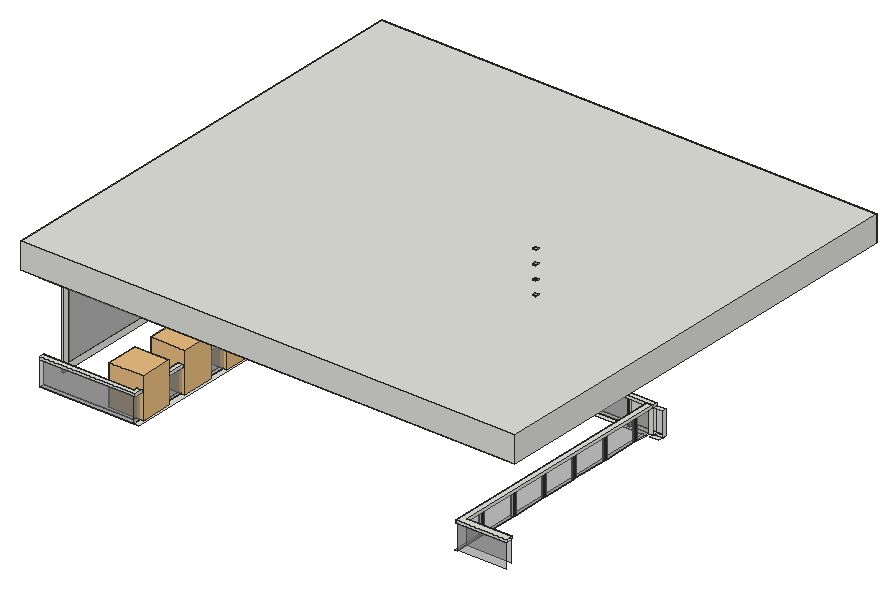
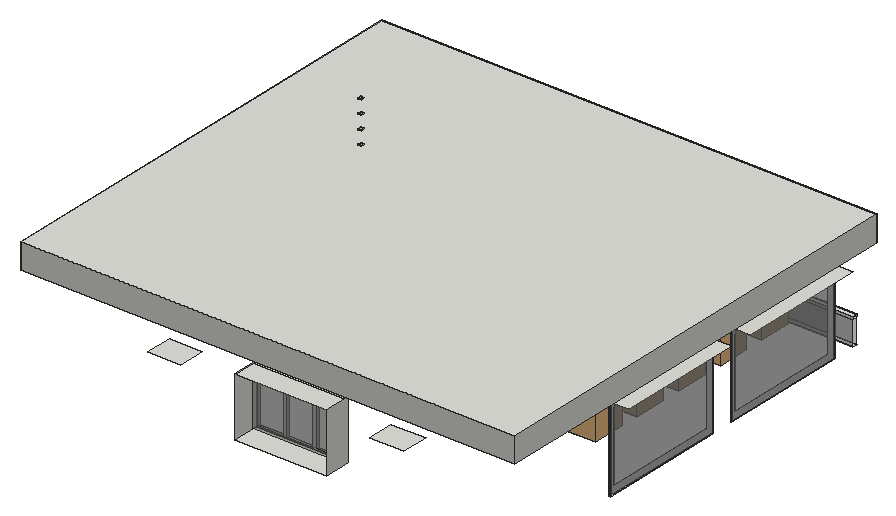
# SketchUp Ruby script. Lengths in inches.
U = 1.inch
M = Sketchup.active_model
def pt(a) = Geom::Point3d.new(a.map { |v| v * U })
def face(e, loops, mat)
  f = e.add_face(loops[0].map { |a| pt(a) })
  loops[1..].each { |l| e.add_face(l.map { |a| pt(a) }).erase! }
  f.material = f.back_material = mat if mat
  f
end
# faces: each face lists its corners as indices into pts; further lists are holes
def faces(e, pts, list, mat = nil) = list.each { |f| face(e, (f[0].is_a?(Array) ? f : [f]).map { |l| l.map { |i| pts[i] } }, mat) }
# xy, xz, yz: faces in a plane at the given z, y or x. An outline is a flat list of corners, or four numbers for a rectangle; further outlines are holes
def ring(l) = l.size == 4 ? [[l[0], l[1]], [l[2], l[1]], [l[2], l[3]], [l[0], l[3]]] : l.each_slice(2).to_a
def flat(e, list, mat, &to3) = list.each { |f| face(e, (f[0].is_a?(Array) ? f : [f]).map { |l| ring(l).map { |u, v| to3.(u, v) } }, mat) }
def xy(e, z, list, mat = nil) = flat(e, list, mat) { |x, y| [x, y, z] }
def xz(e, y, list, mat = nil) = flat(e, list, mat) { |x, z| [x, y, z] }
def yz(e, x, list, mat = nil) = flat(e, list, mat) { |y, z| [x, y, z] }
def lines(e, pts, list) = list.each { |a, b| e.add_line(pt(pts[a]), pt(pts[b])) }
# prism: a flat outline (further loops are holes) pulled along v
def prism(e, loops, v, mat = nil)
  f = face(e, loops, mat); d = Geom::Vector3d.new(v.map { |x| x * U })
  f.pushpull(f.normal.samedirection?(d) ? d.length : -d.length)
end
def box(e, o, s, mat = nil) = prism(e, [[o, [o[0] + s[0], o[1], o[2]], [o[0] + s[0], o[1] + s[1], o[2]], [o[0], o[1] + s[1], o[2]]]], [0, 0, s[2]], mat)
def at(x, y, z, deg = 0) = Geom::Transformation.translation(pt([x, y, z])) * Geom::Transformation.rotation(ORIGIN, Z_AXIS, deg.degrees)
def axes(o, x, y, z) = Geom::Transformation.new([*x, 0, *y, 0, *z, 0, *pt(o).to_a, 1])
def part(name) = M.definitions.add(name)
# library, detail: a bought-in or finely detailed component or shape, given as its bounding box
def library(name, o, s) = part(name).tap { |d| box(d.entities, o, s) }
def detail(e, o, s) = box(e.add_group.entities, o, s)
def put(e, d, t, mat = nil) = e.add_instance(d, t).tap { |i| i.material = mat if mat }
def group(e, t, mat = nil) = e.add_group.tap { |g| g.transformation = t; g.material = mat if mat }.entities
root = M.entities
M.materials.add("Generic").color = [229, 227, 174]
M.materials.add("[Translucent Glass Gray]").color = [128, 128, 128]
M.materials["[Translucent Glass Gray]"].alpha = 0.5
M.materials.add("[Wood Board Cork]").color = [181, 169, 96]
M.materials["[Wood Board Cork]"].alpha = 0.67
c1 = library("Flora+17",[-57.52,158.6,-38.64],[66.99,62.88,77.28])
c2 = part("Group\#2")
xy(c2.entities,0,[[0,0,3,296.5625]])
xy(c2.entities,195.1875,[[0,0,3,296.5625]])
xz(c2.entities,0,[[0,0,3,195.1875]])
xz(c2.entities,296.5625,[[0,0,3,195.1875]])
yz(c2.entities,0,[[0,0,296.5625,195.1875]],"[Translucent Glass Gray]")
yz(c2.entities,3,[[[0,0,296.5625,195.1875],[14.23,14.23,282.34,180.96]]])
yz(c2.entities,3,[[14.23,14.23,282.34,180.96]],"[Translucent Glass Gray]")
c3 = library("Tlon Light 450 Ceiling 152 006",[-8.86,-8.86,-3.78],[17.72,17.72,3.56])
xy(root,231.375,[[45.5625,0,45.5625,11.0625,253.5,11.0625,253.5,562.3125,1038.97,562.3125,1018.75,562.1,1018.84,553.25,966.1875,553.25,966.1875,549.9375,961.1875,549.9375,961.1875,553.25,853.5625,553.25,853.5625,549.9375,848.5625,549.9375,848.5625,553.25,740.9375,553.25,740.9375,549.9375,735.9375,549.9375,735.9375,553.25,609.5,553.25,609.5,549.9375,604.5,549.9375,604.5,553.25,478.0625,553.25,478.0625,549.9375,473.0625,549.9375,473.0625,553.25,346.625,553.25,346.625,549.9375,341.625,549.9375,341.625,553.25,261.0625,553.25,261.0625,512.6,264.375,512.6,264.375,506.23,261.0625,506.23,261.0625,386.1875,264.375,386.1875,264.375,379.8125,261.0625,379.8125,261.0625,279.4375,264.375,279.4375,264.375,273.0625,261.0625,273.0625,261.0625,172.6875,264.375,172.6875,264.375,166.3125,261.0625,166.3125,261.0625,65.9375,264.375,65.9375,264.375,59.5625,261.0625,59.5625,261.0625,0],[261.0625,0,261.0625,59.5625,264.375,59.5625,264.375,65.9375,261.0625,65.9375,261.0625,166.3125,264.375,166.3125,264.375,172.6875,261.0625,172.6875,261.0625,273.0625,264.375,273.0625,264.375,279.4375,261.0625,279.4375,261.0625,379.8125,264.375,379.8125,264.375,386.1875,261.0625,386.1875,261.0625,506.23,264.375,506.23,264.375,512.6,261.0625,512.6,261.0625,553.25,341.625,553.25,341.625,549.9375,346.625,549.9375,346.625,553.25,473.0625,553.25,473.0625,549.9375,478.0625,549.9375,478.0625,553.25,604.5,553.25,604.5,549.9375,609.5,549.9375,609.5,553.25,735.9375,553.25,735.9375,549.9375,740.9375,549.9375,740.9375,553.25,848.5625,553.25,848.5625,549.9375,853.5625,549.9375,853.5625,553.25,961.1875,553.25,961.1875,549.9375,966.1875,549.9375,966.1875,553.25,1018.84,553.25,1018.84,553.04,1038.97,553.25,1038.97,542.9375,1018.875,542.9375,1018.875,549.9375,1010.375,549.9375,1010.375,542.9375,274.125,542.9375,274.125,0],[1003,0,1010.375,0,1010.375,67.5,1005.0625,67.5,1005.0625,73.0625,1010.375,73.0625,1010.375,159.625,1005.0625,159.625,1005.0625,165.1875,1010.375,165.1875,1010.375,247.3125,1005.0625,247.3125,1005.0625,252.875,1010.375,252.875,1010.375,335,1005.0625,335,1005.0625,340.5625,1010.375,340.5625,1010.375,422.6875,1005.0625,422.6875,1005.0625,428.25,1010.375,428.25,1010.375,510.375,1005.0625,510.375,1005.0625,515.9375,1010.375,515.9375,1010.375,542.9375,1003,542.9375],[1018.84,553.04,1018.84,553.25,1038.97,553.25],[1018.84,553.25,1018.75,562.1,1038.97,562.3125,1038.97,553.25],
  [1038.97,553.25,1038.97,562.3125,1039.0625,553.25]])
xy(root,279.55,[[434.63,980.0625,646.76,1041.5]])
xy(root,287.4375,[[45.5625,0,261.0625,0,261.0625,59.5625,264.375,59.5625,264.375,65.9375,261.0625,65.9375,261.0625,166.3125,264.375,166.3125,264.375,172.6875,261.0625,172.6875,261.0625,273.0625,264.375,273.0625,264.375,279.4375,261.0625,279.4375,261.0625,379.8125,264.375,379.8125,264.375,386.1875,261.0625,386.1875,261.0625,506.23,264.375,506.23,264.375,512.6,261.0625,512.6,261.0625,553.25,341.625,553.25,341.625,549.9375,346.625,549.9375,346.625,553.25,473.0625,553.25,473.0625,549.9375,478.0625,549.9375,478.0625,553.25,604.5,553.25,604.5,549.9375,609.5,549.9375,609.5,553.25,735.9375,553.25,735.9375,549.9375,740.9375,549.9375,740.9375,553.25,848.5625,553.25,848.5625,549.9375,853.5625,549.9375,853.5625,553.25,961.1875,553.25,961.1875,549.9375,966.1875,549.9375,966.1875,553.25,1018.84,553.25,1018.78,558.99,1018.75,562.1,1018.875,562.1,1018.875,562.3125,253.5,562.3125,253.5,11.0625,45.5625,11.0625],[261.0625,0,264.375,59.5625],[1005.0625,0,1010.375,67.5],[1010.375,0,1010.375,67.5,1005.0625,67.5,1005.0625,73.0625,1010.375,73.0625,1010.375,159.625,1005.0625,159.625,1005.0625,165.1875,1010.375,165.1875,1010.375,247.3125,1005.0625,247.3125,1005.0625,252.875,1010.375,252.875,1010.375,335,1005.0625,335,1005.0625,340.5625,1010.375,340.5625,1010.375,422.6875,1005.0625,422.6875,1005.0625,428.25,1010.375,428.25,1010.375,510.375,1005.0625,510.375,1005.0625,515.9375,1010.375,515.9375,1010.375,549.9375,1018.875,549.9375,1018.875,15.375,1122.5625,15.375,1122.5625,0],[261.0625,65.9375,264.375,166.3125],
  [1005.0625,73.0625,1010.375,159.625],[1005.0625,165.1875,1010.375,247.3125],[261.0625,172.6875,264.375,273.0625],[1005.0625,252.875,1010.375,335],[261.0625,279.4375,264.375,379.8125],
  [1005.0625,340.5625,1010.375,422.6875],[261.0625,386.1875,264.375,506.23],[1005.0625,428.25,1010.375,510.375],[261.0625,512.6,264.375,549.9375],[1005.0625,515.9375,1010.375,549.9375],
  [261.0625,549.9375,341.625,553.25],[346.625,549.9375,473.0625,553.25],[478.0625,549.9375,604.5,553.25],[609.5,549.9375,735.9375,553.25],[740.9375,549.9375,848.5625,553.25],
  [853.5625,549.9375,961.1875,553.25],[966.1875,549.9375,1018.875,549.9375,1018.875,553.04,1018.84,553.04,1018.84,553.25,966.1875,553.25],[1018.84,553.04,1018.875,553.25],[1018.875,553.04,1039.0625,553.25,1038.97,562.3125,1018.875,562.3125],[1018.84,553.25,1018.875,553.25,1018.875,558.99,1018.78,558.99],
  [1018.78,558.99,1018.875,558.99,1018.875,562.1,1018.75,562.1]])
xy(root,293.625,[[45.5625,0,264.375,0,264.375,549.9375,1018.875,549.9375,1018.875,562.3125,253.5,562.3125,253.5,11.0625,45.5625,11.0625],[1005.0625,0,1122.5625,0,1122.5625,15.375,1018.875,15.375,1018.875,549.9375,1005.0625,549.9375]])
xy(root,392.0625,[[771.78,980.0625,847.11,1041.5]])
xy(root,394.04,[[255.99,980.0625,335.28,1041.5]])
xy(root,416.17,[[434.63,980.0625,646.76,1041.5]])
xy(root,426.5625,[[0,67.54,45.5625,364.1],[0,417.04,45.5625,713.6]])
xy(root,457.375,[[[45.5625,0,45.5625,752.375,1014.875,752.375,1014.875,796.5,1122.5625,796.5,1122.5625,0],[171.79,126.23,996.33,500.33]],[193.51,770,216.14,980.0625],[282.08,770,304.7,980.0625],[370.64,770,393.26,980.0625],[459.2,770,481.83,980.0625],
  [547.76,770,570.39,980.0625],[636.33,770,658.95,980.0625],[724.89,770,747.51,980.0625],[813.45,770,836.08,980.0625],[902.01,770,924.64,980.0625]],"Generic")
xy(root,469.625,[[223.7,160.52,308.39,485.02],[422.95,160.52,507.64,485.02],[622.2,160.52,706.89,485.02],[821.45,160.52,906.14,485.02]],"Generic")
xy(root,483.5625,[[[171.79,126.23,996.33,500.33],[223.7,160.52,308.39,485.02],[422.95,160.52,507.64,485.02],[622.2,160.52,706.89,485.02],[821.45,160.52,906.14,485.02]],[175.5625,752.375,175.5625,980.0625,193.51,980.0625,193.51,770,216.14,770,216.14,980.0625,282.08,980.0625,282.08,770,304.7,770,304.7,980.0625,370.64,980.0625,370.64,770,393.26,770,393.26,980.0625,459.2,980.0625,459.2,770,481.83,770,481.83,980.0625,547.76,980.0625,547.76,770,570.39,770,570.39,980.0625,636.33,980.0625,636.33,770,658.95,770,658.95,980.0625,724.89,980.0625,724.89,770,747.51,770,747.51,980.0625,813.45,980.0625,813.45,770,836.08,770,836.08,980.0625,902.01,980.0625,902.01,770,924.64,770,924.64,980.0625,952.125,980.0625,952.125,752.375]],"Generic")
xy(root,516.29,[[0,0,1142.0625,1041.5]])
xz(root,0,[[45.5625,287.4375,264.375,293.625],[1005.0625,287.4375,1122.5625,293.625],[0,457.375,1142.0625,516.29]])
xz(root,0,[[45.5625,231.375,261.0625,287.4375],[1010.375,231.375,1122.5625,287.4375]],"[Translucent Glass Gray]")
xz(root,11.0625,[[45.5625,287.4375,253.5,293.625]])
xz(root,11.0625,[[45.5625,231.375,253.5,287.4375]],"[Translucent Glass Gray]")
xz(root,15.375,[[1018.875,287.4375,1122.5625,293.625]])
xz(root,15.375,[[1018.875,237.375,1122.5625,287.4375]],"[Translucent Glass Gray]")
xz(root,59.5625,[[261.0625,231.375,264.375,287.4375]])
xz(root,65.9375,[[261.0625,231.375,264.375,287.4375]])
xz(root,67.5,[[1005.0625,231.375,1010.375,287.4375]])
xz(root,73.0625,[[1005.0625,231.375,1010.375,287.4375]])
xz(root,126.23,[[171.79,457.375,996.33,483.5625]])
xz(root,159.625,[[1005.0625,231.375,1010.375,287.4375]])
xz(root,160.52,[[223.7,469.625,308.39,483.5625],[422.95,469.625,507.64,483.5625],[622.2,469.625,706.89,483.5625],[821.45,469.625,906.14,483.5625]])
xz(root,165.1875,[[1005.0625,231.375,1010.375,287.4375]])
xz(root,166.3125,[[261.0625,231.375,264.375,287.4375]])
xz(root,172.6875,[[261.0625,231.375,264.375,287.4375]])
xz(root,247.3125,[[1005.0625,231.375,1010.375,287.4375]])
xz(root,252.875,[[1005.0625,231.375,1010.375,287.4375]])
xz(root,273.0625,[[261.0625,231.375,264.375,287.4375]])
xz(root,279.4375,[[261.0625,231.375,264.375,287.4375]])
xz(root,335,[[1005.0625,231.375,1010.375,287.4375]])
xz(root,340.5625,[[1005.0625,231.375,1010.375,287.4375]])
xz(root,379.8125,[[261.0625,231.375,264.375,287.4375]])
xz(root,386.1875,[[261.0625,231.375,264.375,287.4375]])
xz(root,422.6875,[[1005.0625,231.375,1010.375,287.4375]])
xz(root,428.25,[[1005.0625,231.375,1010.375,287.4375]])
xz(root,485.02,[[223.7,469.625,308.39,483.5625],[422.95,469.625,507.64,483.5625],[622.2,469.625,706.89,483.5625],[821.45,469.625,906.14,483.5625]])
xz(root,500.33,[[171.79,457.375,996.33,483.5625]],"Generic")
xz(root,506.23,[[261.0625,231.375,264.375,287.4375]])
xz(root,510.375,[[1005.0625,231.375,1010.375,287.4375]])
xz(root,512.6,[[261.0625,231.375,264.375,287.4375]])
xz(root,515.9375,[[1005.0625,231.375,1010.375,287.4375]])
xz(root,549.9375,[[341.625,231.375,346.625,287.4375],[473.0625,231.375,478.0625,287.4375],[604.5,231.375,609.5,287.4375],[735.9375,231.375,740.9375,287.4375],[848.5625,231.375,853.5625,287.4375],
  [961.1875,231.375,966.1875,287.4375],[1010.375,231.375,1018.875,287.4375],[264.375,287.4375,1005.0625,293.625],[1005.0625,287.4375,1018.875,293.625]])
xz(root,553.25,[[261.0625,231.375,341.625,287.4375],[346.625,231.375,473.0625,287.4375],[478.0625,231.375,604.5,287.4375],[609.5,231.375,735.9375,287.4375],[740.9375,231.375,848.5625,287.4375],
  [853.5625,231.375,961.1875,287.4375]],"[Translucent Glass Gray]")
xz(root,562.3125,[[253.5,287.4375,1018.875,293.625]])
xz(root,562.3125,[[253.5,231.375,1038.97,287.4375]],"[Translucent Glass Gray]")
xz(root,752.375,[[175.5625,457.375,952.125,483.5625]])
xz(root,770,[[193.51,457.375,216.14,483.5625],[282.08,457.375,304.7,483.5625],[370.64,457.375,393.26,483.5625],[459.2,457.375,481.83,483.5625],[547.76,457.375,570.39,483.5625],
  [636.33,457.375,658.95,483.5625],[724.89,457.375,747.51,483.5625],[813.45,457.375,836.08,483.5625],[902.01,457.375,924.64,483.5625]])
xz(root,980.0625,[[175.5625,457.375,193.51,483.5625]])
xz(root,1041.5,[[0,457.375,1142.0625,516.29]])
yz(root,0,[[0,457.375,1041.5,516.29]])
yz(root,171.79,[[126.23,457.375,500.33,483.5625]],"Generic")
yz(root,193.51,[[770,457.375,980.0625,483.5625]])
yz(root,216.14,[[770,457.375,980.0625,483.5625]],"Generic")
yz(root,223.7,[[160.52,469.625,485.02,483.5625]],"Generic")
yz(root,253.5,[[11.0625,287.4375,562.3125,293.625]])
yz(root,253.5,[[11.0625,231.375,562.3125,287.4375]],"[Translucent Glass Gray]")
yz(root,261.0625,[[0,231.375,59.5625,287.4375],[65.9375,231.375,166.3125,287.4375],[172.6875,231.375,273.0625,287.4375],[279.4375,231.375,379.8125,287.4375],[386.1875,231.375,506.23,287.4375],
  [512.6,231.375,553.25,287.4375]],"[Translucent Glass Gray]")
yz(root,264.375,[[59.5625,231.375,65.9375,287.4375],[166.3125,231.375,172.6875,287.4375],[273.0625,231.375,279.4375,287.4375],[379.8125,231.375,386.1875,287.4375],[506.23,231.375,512.6,287.4375],
  [0,287.4375,549.9375,293.625]])
yz(root,282.08,[[770,457.375,980.0625,483.5625]],"Generic")
yz(root,304.7,[[770,457.375,980.0625,483.5625]],"Generic")
yz(root,308.39,[[160.52,469.625,485.02,483.5625]],"Generic")
yz(root,341.625,[[549.9375,231.375,553.25,287.4375]])
yz(root,346.625,[[549.9375,231.375,553.25,287.4375]])
yz(root,370.64,[[770,457.375,980.0625,483.5625]],"Generic")
yz(root,393.26,[[770,457.375,980.0625,483.5625]],"Generic")
yz(root,422.95,[[160.52,469.625,485.02,483.5625]],"Generic")
yz(root,434.63,[[980.0625,279.55,1041.5,416.17]])
yz(root,459.2,[[770,457.375,980.0625,483.5625]],"Generic")
yz(root,473.0625,[[549.9375,231.375,553.25,287.4375]])
yz(root,478.0625,[[549.9375,231.375,553.25,287.4375]])
yz(root,481.83,[[770,457.375,980.0625,483.5625]],"Generic")
yz(root,507.64,[[160.52,469.625,485.02,483.5625]],"Generic")
yz(root,547.76,[[770,457.375,980.0625,483.5625]],"Generic")
yz(root,570.39,[[770,457.375,980.0625,483.5625]],"Generic")
yz(root,604.5,[[549.9375,231.375,553.25,287.4375]])
yz(root,609.5,[[549.9375,231.375,553.25,287.4375]])
yz(root,622.2,[[160.52,469.625,485.02,483.5625]],"Generic")
yz(root,636.33,[[770,457.375,980.0625,483.5625]],"Generic")
yz(root,646.76,[[980.0625,279.55,1041.5,416.17]])
yz(root,658.95,[[770,457.375,980.0625,483.5625]],"Generic")
yz(root,706.89,[[160.52,469.625,485.02,483.5625]],"Generic")
yz(root,724.89,[[770,457.375,980.0625,483.5625]],"Generic")
yz(root,735.9375,[[549.9375,231.375,553.25,287.4375]])
yz(root,740.9375,[[549.9375,231.375,553.25,287.4375]])
yz(root,747.51,[[770,457.375,980.0625,483.5625]],"Generic")
yz(root,813.45,[[770,457.375,980.0625,483.5625]],"Generic")
yz(root,821.45,[[160.52,469.625,485.02,483.5625]],"Generic")
yz(root,836.08,[[770,457.375,980.0625,483.5625]],"Generic")
yz(root,848.5625,[[549.9375,231.375,553.25,287.4375]])
yz(root,853.5625,[[549.9375,231.375,553.25,287.4375]])
yz(root,902.01,[[770,457.375,980.0625,483.5625]],"Generic")
yz(root,906.14,[[160.52,469.625,485.02,483.5625]],"Generic")
yz(root,924.64,[[770,457.375,980.0625,483.5625]],"Generic")
yz(root,961.1875,[[549.9375,231.375,553.25,287.4375]])
yz(root,966.1875,[[549.9375,231.375,553.25,287.4375]])
yz(root,996.33,[[126.23,457.375,500.33,483.5625]],"Generic")
yz(root,1005.0625,[[67.5,231.375,73.0625,287.4375],[159.625,231.375,165.1875,287.4375],[247.3125,231.375,252.875,287.4375],[335,231.375,340.5625,287.4375],[422.6875,231.375,428.25,287.4375],
  [510.375,231.375,515.9375,287.4375],[0,287.4375,549.9375,293.625]])
yz(root,1010.375,[[0,231.375,67.5,287.4375],[73.0625,231.375,159.625,287.4375],[165.1875,231.375,247.3125,287.4375],[252.875,231.375,335,287.4375],[340.5625,231.375,422.6875,287.4375],
  [428.25,231.375,510.375,287.4375],[515.9375,231.375,549.9375,287.4375]],"[Translucent Glass Gray]")
yz(root,1018.875,[[15.375,287.4375,549.9375,293.625],[549.9375,287.4375,562.3125,293.625]])
yz(root,1142.0625,[[0,457.375,1041.5,516.29]])
p = [[1038.97,562.3125,231.375],[1039.0625,553.25,231.375],[1039.0625,553.25,287.4375],[1038.97,562.3125,287.4375],[1018.75,562.1,287.4375],[1018.75,562.1,231.375]]
faces(root,p,[[0,1,2,3]])
lines(root,p,[[4,5]])
put(root,c1,axes([257.04,-169.3,277.36],[1.19,0,0],[0,1.19,0],[0,0,1.19]))
put(root,c1,axes([257.04,-49.43,277.36],[1.19,0,0],[0,1.19,0],[0,0,1.19]))
put(root,c1,axes([257.04,70.45,277.36],[1.19,0,0],[0,1.19,0],[0,0,1.19]))
put(root,c1,axes([257.04,190.32,277.36],[1.19,0,0],[0,1.19,0],[0,0,1.19]))
put(root,c1,axes([257.04,310.2,277.36],[1.19,0,0],[0,1.19,0],[0,0,1.19]))
put(root,c2,at(42.5625,417.04,231.375))
put(root,c2,at(42.5625,67.54,231.375))
g1 = group(root,at(434.63,980.0625,279.55))
xy(g1,0,[[0,0,212.125,9.0625]])
xy(g1,7.45,[[7.45,0,68.22,6.0625],[75.68,0,136.45,6.0625],[143.9,0,204.67,6.0625]])
xy(g1,129.17,[[7.45,0,68.22,6.0625],[75.68,0,136.45,6.0625],[143.9,0,204.67,6.0625]])
xy(g1,136.625,[[0,0,212.125,9.0625]])
xz(g1,0,[[[0,0,212.125,136.625],[75.68,7.45,136.45,129.17],[143.9,7.45,204.67,129.17],[7.45,7.45,68.22,129.17]]],"[Wood Board Cork]")
xz(g1,6.0625,[[7.45,7.45,68.22,129.17],[75.68,7.45,136.45,129.17],[143.9,7.45,204.67,129.17]],"[Translucent Glass Gray]")
xz(g1,9.0625,[[0,0,212.125,136.625]],"[Translucent Glass Gray]")
yz(g1,0,[[0,0,9.0625,136.625]])
yz(g1,7.45,[[0,7.45,6.0625,129.17]])
yz(g1,68.22,[[0,7.45,6.0625,129.17]])
yz(g1,75.68,[[0,7.45,6.0625,129.17]])
yz(g1,136.45,[[0,7.45,6.0625,129.17]])
yz(g1,143.9,[[0,7.45,6.0625,129.17]])
yz(g1,204.67,[[0,7.45,6.0625,129.17]])
yz(g1,212.125,[[0,0,9.0625,136.625]])
put(root,c3,at(986.77,593.18,459.375))
put(root,c3,at(895.4,593.18,459.375))
put(root,c3,at(804.02,593.18,459.375))
put(root,c3,at(712.65,593.18,459.375))
put(root,c3,at(621.27,593.18,459.375))
put(root,c3,at(529.9,593.18,459.375))
put(root,c3,at(438.52,593.18,459.375))
put(root,c3,at(347.15,593.18,459.375))
put(root,c3,at(255.77,593.18,459.375))
put(root,c3,at(164.4,593.18,459.375))
put(root,c3,axes([866.93,415.36,470.53],[0.44,0,0],[0,0.44,0],[0,0,0.44]))
put(root,c3,axes([866.93,350.24,470.53],[0.44,0,0],[0,0.44,0],[0,0,0.44]))
put(root,c3,axes([866.93,297.74,470.53],[0.44,0,0],[0,0.44,0],[0,0,0.44]))
put(root,c3,axes([866.93,245.24,470.53],[0.44,0,0],[0,0.44,0],[0,0,0.44]))
put(root,c3,axes([866.93,192.74,470.53],[0.44,0,0],[0,0.44,0],[0,0,0.44]))
put(root,c3,axes([866.93,140.24,470.53],[0.44,0,0],[0,0.44,0],[0,0,0.44]))
put(root,c3,axes([670.99,192.74,470.53],[0.44,0,0],[0,0.44,0],[0,0,0.44]))
put(root,c3,axes([670.99,415.36,470.53],[0.44,0,0],[0,0.44,0],[0,0,0.44]))
put(root,c3,axes([670.99,245.24,470.53],[0.44,0,0],[0,0.44,0],[0,0,0.44]))
put(root,c3,axes([670.99,297.74,470.53],[0.44,0,0],[0,0.44,0],[0,0,0.44]))
put(root,c3,axes([670.99,350.24,470.53],[0.44,0,0],[0,0.44,0],[0,0,0.44]))
put(root,c3,axes([466.18,415.36,470.53],[0.44,0,0],[0,0.44,0],[0,0,0.44]))
put(root,c3,axes([466.18,297.74,470.53],[0.44,0,0],[0,0.44,0],[0,0,0.44]))
put(root,c3,axes([466.18,350.24,470.53],[0.44,0,0],[0,0.44,0],[0,0,0.44]))
put(root,c3,axes([466.18,245.24,470.53],[0.44,0,0],[0,0.44,0],[0,0,0.44]))
put(root,c3,axes([466.18,192.74,470.53],[0.44,0,0],[0,0.44,0],[0,0,0.44]))
put(root,c3,axes([267.18,245.24,470.53],[0.44,0,0],[0,0.44,0],[0,0,0.44]))
put(root,c3,axes([267.18,350.24,470.53],[0.44,0,0],[0,0.44,0],[0,0,0.44]))
put(root,c3,axes([267.18,415.36,470.53],[0.44,0,0],[0,0.44,0],[0,0,0.44]))
put(root,c3,axes([267.18,297.74,470.53],[0.44,0,0],[0,0.44,0],[0,0,0.44]))
put(root,c3,axes([267.18,192.74,470.53],[0.44,0,0],[0,0.44,0],[0,0,0.44]))
put(root,c3,axes([866.93,402.74,502.41],[0.44,0,0],[0,0.44,0],[0,0,0.44]))
put(root,c3,axes([866.93,402.74,534.28],[0.44,0,0],[0,0.44,0],[0,0,0.44]))
put(root,c3,axes([866.93,402.74,566.16],[0.44,0,0],[0,0.44,0],[0,0,0.44]))
put(root,c3,axes([866.93,402.74,598.03],[0.44,0,0],[0,0.44,0],[0,0,0.44]))
put(root,c3,axes([866.93,402.74,629.91],[0.44,0,0],[0,0.44,0],[0,0,0.44]))
